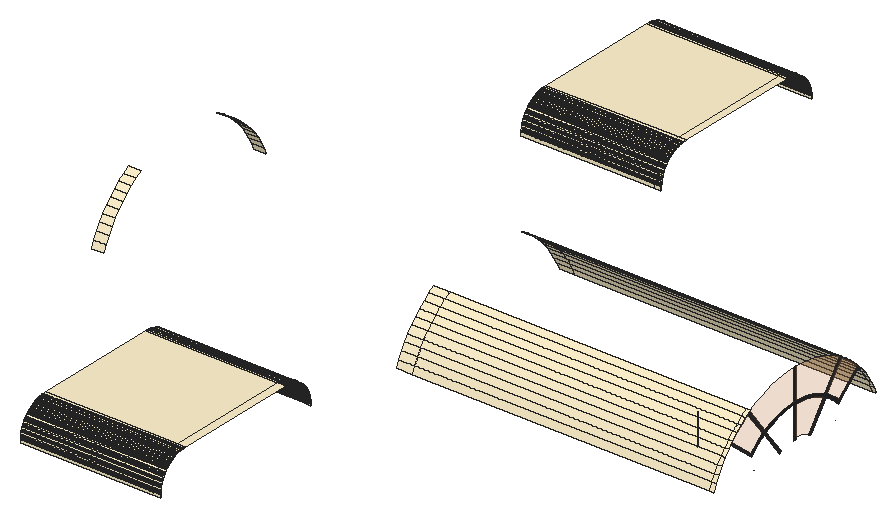
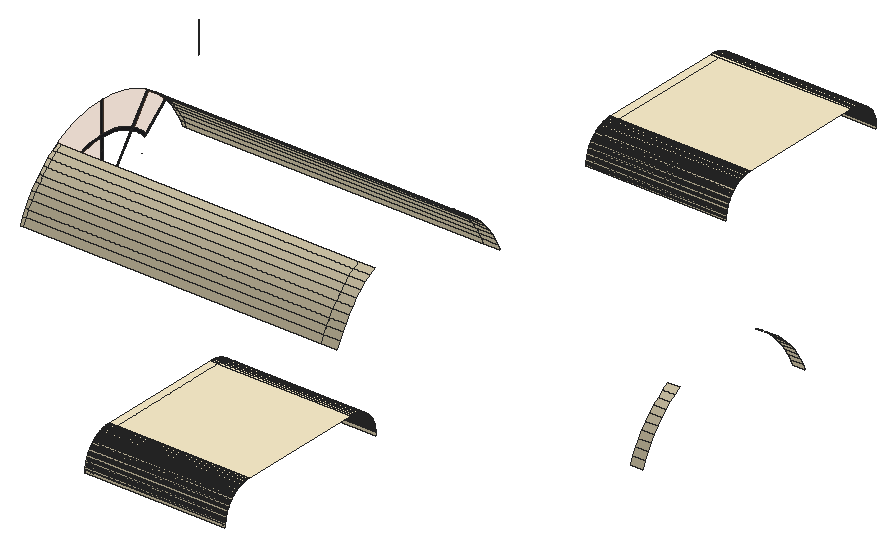
# SketchUp Ruby script. Lengths in inches.
U = 1.inch
M = Sketchup.active_model
def pt(a) = Geom::Point3d.new(a.map { |v| v * U })
def face(e, loops, mat)
  f = e.add_face(loops[0].map { |a| pt(a) })
  loops[1..].each { |l| e.add_face(l.map { |a| pt(a) }).erase! }
  f.material = f.back_material = mat if mat
  f
end
# faces: each face lists its corners as indices into pts; further lists are holes
def faces(e, pts, list, mat = nil) = list.each { |f| face(e, (f[0].is_a?(Array) ? f : [f]).map { |l| l.map { |i| pts[i] } }, mat) }
# xy, xz, yz: faces in a plane at the given z, y or x. An outline is a flat list of corners, or four numbers for a rectangle; further outlines are holes
def ring(l) = l.size == 4 ? [[l[0], l[1]], [l[2], l[1]], [l[2], l[3]], [l[0], l[3]]] : l.each_slice(2).to_a
def flat(e, list, mat, &to3) = list.each { |f| face(e, (f[0].is_a?(Array) ? f : [f]).map { |l| ring(l).map { |u, v| to3.(u, v) } }, mat) }
def xy(e, z, list, mat = nil) = flat(e, list, mat) { |x, y| [x, y, z] }
def xz(e, y, list, mat = nil) = flat(e, list, mat) { |x, z| [x, y, z] }
def yz(e, x, list, mat = nil) = flat(e, list, mat) { |y, z| [x, y, z] }
def lines(e, pts, list) = list.each { |a, b| e.add_line(pt(pts[a]), pt(pts[b])) }
# prism: a flat outline (further loops are holes) pulled along v
def prism(e, loops, v, mat = nil)
  f = face(e, loops, mat); d = Geom::Vector3d.new(v.map { |x| x * U })
  f.pushpull(f.normal.samedirection?(d) ? d.length : -d.length)
end
def box(e, o, s, mat = nil) = prism(e, [[o, [o[0] + s[0], o[1], o[2]], [o[0] + s[0], o[1] + s[1], o[2]], [o[0], o[1] + s[1], o[2]]]], [0, 0, s[2]], mat)
def at(x, y, z, deg = 0) = Geom::Transformation.translation(pt([x, y, z])) * Geom::Transformation.rotation(ORIGIN, Z_AXIS, deg.degrees)
def axes(o, x, y, z) = Geom::Transformation.new([*x, 0, *y, 0, *z, 0, *pt(o).to_a, 1])
def part(name) = M.definitions.add(name)
# library, detail: a bought-in or finely detailed component or shape, given as its bounding box
def library(name, o, s) = part(name).tap { |d| box(d.entities, o, s) }
def detail(e, o, s) = box(e.add_group.entities, o, s)
def put(e, d, t, mat = nil) = e.add_instance(d, t).tap { |i| i.material = mat if mat }
def group(e, t, mat = nil) = e.add_group.tap { |g| g.transformation = t; g.material = mat if mat }.entities
root = M.entities
M.materials.add("D01_Frost_White").color = [255, 242, 206]
M.materials.add("Glass_Safety_01").color = [244, 153, 81]
M.materials["Glass_Safety_01"].alpha = 0.25
M.materials.add("ThomThom - Buttons1").color = [48, 49, 53]
M.materials.add("ThomThom - Buttons2").color = [40, 40, 43]
xy(root,342,[[144.65,88.1,246,90],[246,88.1,252,90],[144.65,90,246,186],[246,90,252,186],[144.65,186,246,187.16],
  [246,186,252,187.16],[144.65,567.32,246,570],[246,567.32,252,570],[144.65,570,246,666],[246,570,252,666],
  [144.65,666,246,667.87],[246,666,252,667.87]],"D01_Frost_White")
xz(root,66,[[144.65,318,246,319.9],[246,318,252,319.9]],"D01_Frost_White")
xz(root,210,[[144.65,318,246,319.16],[246,318,252,319.16]],"D01_Frost_White")
xz(root,546,[[144.65,318,246,320.68],[246,318,252,320.68]],"D01_Frost_White")
xz(root,690,[[144.65,318,246,319.87],[246,318,252,319.87]],"D01_Frost_White")
yz(root,252,[[66,318,66,319.9,65.98,319.53,65.98,318.76],[210,318,210.01,318.76,210,319.16],[546,318,546,320.68,545.98,320.3,545.96,319.53,545.97,318.77],[690,318,690.02,318.76,690.01,319.53,690,319.87],[88.1,342,90,342,89.24,342.02,88.47,342.02],
  [186,342,187.16,342,186.76,342.01],[567.32,342,570,342,569.23,342.03,568.47,342.04,567.7,342.02],[666,342,667.87,342,667.53,342.01,666.76,342.02]],"D01_Frost_White")
yz(root,489,[[338.87,299.58,338.96,299.71,338.92,299.66],[417.13,299.58,417.08,299.66,417.04,299.71],[390.99,301.79,405.47,321.06,403.79,321.96,400.3125,323.54,396.74,324.89,393.09,325.99,389.375,326.86,385.61,327.49,381.8125,327.86,379,327.95,379,304.66,379.92,304.63,381.82,304.45,383.72,304.15,385.59,303.73,387.43,303.2,389.23,302.55],[419.56,310.51,419.21,310.875,418.48,311.56],[335.88,312.77,338.25,314.99,341.29,317.5,344.5,319.8,347.51,321.68,333.04,340.94,331.13,339.75,326.65,336.53,322.39,333.02,318.36,329.24,317.4,328.21],
  [420.03,312.85,438.53,328.29,437.64,329.24,433.61,333.02,429.35,336.53,424.87,339.75,422.83,341.02,422.26,340.27,408.36,321.76,411.5,319.8,414.71,317.5,417.75,314.99],[349.18,322.6,351.33,323.75,354.92,325.39,358.61,326.78,362.39,327.93,366.23,328.83,370.13,329.47,374.06,329.86,378,329.99,377,329.99,377,353.97,372.48,353.82,366.99,353.28,361.54,352.375,356.16,351.12,350.88,349.51,345.71,347.5625,340.6875,345.28,335.82,342.67,334.65,341.94],[406.68,322.68,421.22,342.02,420.18,342.67,415.3125,345.28,410.29,347.5625,405.12,349.51,399.84,351.12,394.46,352.375,389.01,353.28,383.52,353.82,379,353.97,379,329.99,378,329.99,381.94,329.86,385.87,329.47,389.77,328.83,393.61,327.93,397.39,326.78,401.08,325.39,404.67,323.75]],"Glass_Safety_01")
yz(root,489,[[363.12,300.92,364.82,301.79,350.4,320.99,348.85,320.16,348.72,320.08],[392.69,300.92,407.15,320.16,405.47,321.06,390.99,301.79],[336.36,310.42,336.79,310.875,337.43,311.47,337.32,311.56,336.25,310.51],[334.82,311.7,335.37,312.29,335.88,312.77,317.4,328.21,316.37,327.1],[421.1,311.79,439.55,327.19,438.53,328.29,420.03,312.85,420.63,312.29],
  [347.51,321.68,347.85,321.89,349.18,322.6,334.65,341.94,333.04,340.94],[408.36,321.76,422.26,340.27,422.83,341.02,421.22,342.02,406.68,322.68,408.15,321.89]],"ThomThom - Buttons1")
yz(root,489,[[377,303.66,378,303.6875,379,303.66,379,304.66,378,304.6875,377,304.66],[377,304.66,378,304.6875,379,304.66,379,319.07,378,319.08,377,319.07],[336.25,310.51,337.32,311.56,335.88,312.77,335.37,312.29,334.82,311.7],[419.56,310.51,421.1,311.79,420.63,312.29,420.03,312.85,418.48,311.56,419.21,310.875],[337.43,311.47,339.57,313.49,342.51,315.91,345.61,318.14,348.72,320.08,348.66,320.16,347.51,321.68,344.5,319.8,341.29,317.5,338.25,314.99,335.88,312.77,337.32,311.56],
  [418.48,311.56,420.03,312.85,417.75,314.99,414.71,317.5,411.5,319.8,408.36,321.76,407.15,320.16,410.39,318.14,413.49,315.91,416.43,313.49],[377,319.07,378,319.08,379,319.07,379,327.95,381.8125,327.86,385.61,327.49,389.375,326.86,393.09,325.99,396.74,324.89,400.3125,323.54,403.79,321.96,405.47,321.06,406.68,322.68,404.67,323.75,401.08,325.39,397.39,326.78,393.61,327.93,389.77,328.83,385.87,329.47,381.94,329.86,378,329.99,374.06,329.86,370.13,329.47,366.23,328.83,362.39,327.93,358.61,326.78,354.92,325.39,351.33,323.75,349.18,322.6,350.34,321.06,350.4,320.99,352.21,321.96,355.6875,323.54,359.26,324.89,362.91,325.99,366.625,326.86,370.39,327.49,374.1875,327.86,377,327.95],[348.72,320.08,348.85,320.16,350.4,320.99,350.34,321.06,348.66,320.16],[348.66,320.16,350.34,321.06,349.18,322.6,347.85,321.89,347.51,321.68],[407.15,320.16,408.36,321.76,408.15,321.89,406.68,322.68,405.47,321.06],
  [377,329.99,379,329.99,379,353.97,378,354,377,353.97]],"ThomThom - Buttons2")
yz(root,491,[[282,342,282.07,342.73,282.07,365.93,282,366]],"D01_Frost_White")
p = [[21,302.4,306.86],[21,300.13,301.83],[12,300.13,301.83],[12,302.4,306.86],[258,302.4,306.86],[258,300.13,301.83],
  [246,300.13,301.83],[246,302.4,306.86],[486,302.4,306.86],[486,300.13,301.83],[489,302.4,306.86],[489,300.13,301.83],
  [21,455.87,301.83],[21,453.6,306.86],[12,453.6,306.86],[12,455.87,301.83],[258,455.87,301.83],[258,453.6,306.86],
  [246,453.6,306.86],[246,455.87,301.83],[486,455.87,301.83],[486,453.6,306.86],[489,455.87,301.83],[489,453.6,306.86],
  [21,304.99,311.74],[12,304.99,311.74],[258,304.99,311.74],[246,304.99,311.74],[486,304.99,311.74],[489,304.99,311.74],
  [21,451.01,311.74],[12,451.01,311.74],[258,451.01,311.74],[246,451.01,311.74],[486,451.01,311.74],[489,451.01,311.74],
  [21,307.89,316.43],[12,307.89,316.43],[258,307.89,316.43],[246,307.89,316.43],[486,307.89,316.43],[489,307.89,316.43],
  [21,448.11,316.43],[12,448.11,316.43],[258,448.11,316.43],[246,448.11,316.43],[486,448.11,316.43],[489,448.11,316.43],
  [21,311.1,320.93],[12,311.1,320.93],[258,311.1,320.93],[246,311.1,320.93],[486,311.1,320.93],[489,311.1,320.93],
  [21,444.9,320.93],[12,444.9,320.93],[258,444.9,320.93],[246,444.9,320.93],[486,444.9,320.93],[489,444.9,320.93],
  [246,210,319.16],[246,209.99,319.52],[144.65,209.99,319.52],[144.65,210,319.16],[252,210,319.16],[252,209.99,319.52],
  [246,209.95,320.28],[144.65,209.95,320.28],[252,209.95,320.28],[246,66.02,320.29],[246,66,319.9],[144.65,66,319.9],
  [144.65,66.02,320.29],[252,66.02,320.29],[252,66,319.9],[246,690,319.87],[246,689.98,320.29],[144.65,689.98,320.29],
  [144.65,690,319.87],[252,690,319.87],[252,689.98,320.29],[246,66.07,321.05],[144.65,66.07,321.05],[252,66.07,321.05],
  [246,209.89,321.03],[144.65,209.89,321.03],[252,209.89,321.03],[246,689.93,321.05],[144.65,689.93,321.05],[252,689.93,321.05],
  [246,546.02,321.07],[246,546,320.68],[144.65,546,320.68],[144.65,546.02,321.07],[252,546.02,321.07],[252,546,320.68],
  [21,314.59,325.2],[12,314.59,325.2],[258,314.59,325.2],[246,314.59,325.2],[486,314.59,325.2],[489,314.59,325.2],
  [21,441.41,325.2],[12,441.41,325.2],[258,441.41,325.2],[246,441.41,325.2],[486,441.41,325.2],[489,441.41,325.2],
  [246,66.15,321.81],[144.65,66.15,321.81],[252,66.15,321.81],[246,209.8,321.79],[144.65,209.8,321.79],[252,209.8,321.79],
  [246,689.85,321.81],[144.65,689.85,321.81],[252,689.85,321.81],[246,546.09,321.83],[144.65,546.09,321.83],[252,546.09,321.83],
  [246,66.26,322.5625],[144.65,66.26,322.5625],[252,66.26,322.5625],[246,209.68,322.54],[144.65,209.68,322.54],[252,209.68,322.54],
  [246,546.1875,322.59],[144.65,546.1875,322.59],[252,546.1875,322.59],[246,689.74,322.5625],[144.65,689.74,322.5625],[252,689.74,322.5625],
  [246,209.54,323.29],[144.65,209.54,323.29],[252,209.54,323.29],[246,66.39,323.32],[144.65,66.39,323.32],[252,66.39,323.32],
  [246,546.3125,323.35],[144.65,546.3125,323.35],[252,546.3125,323.35],[246,689.61,323.31],[144.65,689.61,323.31],[252,689.61,323.31],
  [246,66.54,324.0625],[144.65,66.54,324.0625],[252,66.54,324.0625],[246,209.38,324.03],[144.65,209.38,324.03],[252,209.38,324.03],
  [246,546.46,324.1],[144.65,546.46,324.1],[252,546.46,324.1],[246,689.45,324.0625],[144.65,689.45,324.0625],[252,689.45,324.0625],
  [246,209.19,324.77],[144.65,209.19,324.77],[252,209.19,324.77],[246,66.72,324.8],[144.65,66.72,324.8],[252,66.72,324.8],
  [246,546.63,324.85],[144.65,546.63,324.85],[252,546.63,324.85],[246,689.27,324.8],[144.65,689.27,324.8],[252,689.27,324.8],
  [246,66.93,325.54],[144.65,66.93,325.54],[252,66.93,325.54],[246,208.98,325.5],[144.65,208.98,325.5],[252,208.98,325.5],
  [246,546.83,325.59],[144.65,546.83,325.59],[252,546.83,325.59],[246,689.07,325.54],[144.65,689.07,325.54],[252,689.07,325.54],
  [21,318.36,329.24],[12,318.36,329.24],[258,318.36,329.24],[246,318.36,329.24],[486,318.36,329.24],[489,316.37,327.1],
  [489,318.36,329.24],[489,317.4,328.21],[21,437.64,329.24],[12,437.64,329.24],[258,437.64,329.24],[246,437.64,329.24],
  [486,437.64,329.24],[489,438.53,328.29],[489,437.64,329.24],[489,439.55,327.19],[246,67.16,326.27],[144.65,67.16,326.27],
  [252,67.16,326.27],[246,208.75,326.22],[144.65,208.75,326.22],[252,208.75,326.22],[246,688.84,326.27],[144.65,688.84,326.27],
  [252,688.84,326.27],[246,547.05,326.32],[144.65,547.05,326.32],[252,547.05,326.32],[246,208.49,326.93],[144.65,208.49,326.93],
  [252,208.49,326.93],[246,67.41,326.99],[144.65,67.41,326.99],[252,67.41,326.99],[246,547.3,327.05],[144.65,547.3,327.05],
  [252,547.3,327.05],[246,688.58,326.98],[144.65,688.58,326.98],[252,688.58,326.98],[246,208.21,327.64],[144.65,208.21,327.64],
  [252,208.21,327.64],[246,67.6875,327.7],[144.65,67.6875,327.7],[252,67.6875,327.7],[246,547.57,327.77],[144.65,547.57,327.77],
  [252,547.57,327.77],[246,688.31,327.7],[144.65,688.31,327.7],[252,688.31,327.7],[246,207.9,328.33],[144.65,207.9,328.33],
  [252,207.9,328.33],[246,67.99,328.4],[144.65,67.99,328.4],[252,67.99,328.4],[246,688.01,328.4],[144.65,688.01,328.4],
  [252,688.01,328.4],[246,547.87,328.47],[144.65,547.87,328.47],[252,547.87,328.47],[246,207.58,329.02],[144.65,207.58,329.02],
  [252,207.58,329.02],[246,68.3125,329.09],[144.65,68.3125,329.09],[252,68.3125,329.09],[246,687.68,329.09],[144.65,687.68,329.09],
  [252,687.68,329.09],[246,548.1875,329.17],[144.65,548.1875,329.17],[252,548.1875,329.17],[246,207.23,329.7],[144.65,207.23,329.7],
  [252,207.23,329.7],[246,68.66,329.77],[144.65,68.66,329.77],[252,68.66,329.77],[246,687.34,329.77],[144.65,687.34,329.77],
  [252,687.34,329.77],[21,322.39,333.02],[12,322.39,333.02],[258,322.39,333.02],[246,322.39,333.02],[486,322.39,333.02],
  [489,322.39,333.02],[21,433.61,333.02],[12,433.61,333.02],[258,433.61,333.02],[246,433.61,333.02],[486,433.61,333.02],
  [489,433.61,333.02],[246,548.53,329.86],[144.65,548.53,329.86],[252,548.53,329.86],[246,206.86,330.36],[144.65,206.86,330.36],
  [252,206.86,330.36],[246,69.03,330.44],[144.65,69.03,330.44],[252,69.03,330.44],[246,686.97,330.4375],[144.65,686.97,330.4375],
  [252,686.97,330.4375],[246,548.9,330.53],[144.65,548.9,330.53],[252,548.9,330.53],[246,69.42,331.1],[144.65,69.42,331.1],
  [252,69.42,331.1],[246,206.47,331.01],[144.65,206.47,331.01],[252,206.47,331.01],[246,686.58,331.09],[144.65,686.58,331.09],
  [252,686.58,331.09],[246,549.29,331.19],[144.65,549.29,331.19],[252,549.29,331.19],[246,206.05,331.65],[144.65,206.05,331.65],
  [252,206.05,331.65],[246,69.83,331.74],[144.65,69.83,331.74],[252,69.83,331.74],[246,686.17,331.73],[144.65,686.17,331.73],
  [252,686.17,331.73],[246,549.7,331.84],[144.65,549.7,331.84],[252,549.7,331.84],[246,205.62,332.27],[144.65,205.62,332.27],
  [252,205.62,332.27],[246,70.26,332.37],[144.65,70.26,332.37],[252,70.26,332.37],[246,685.73,332.36],[144.65,685.73,332.36],
  [252,685.73,332.36],[246,550.13,332.47],[144.65,550.13,332.47],[252,550.13,332.47],[246,205.17,332.88],[144.65,205.17,332.88],
  [252,205.17,332.88],[246,70.71,332.98],[144.65,70.71,332.98],[252,70.71,332.98],[246,685.28,332.98],[144.65,685.28,332.98],
  [252,685.28,332.98],[246,550.58,333.09],[144.65,550.58,333.09],[252,550.58,333.09],[246,204.69,333.48],[144.65,204.69,333.48],
  [252,204.69,333.48],[246,71.1875,333.58],[144.65,71.1875,333.58],[252,71.1875,333.58],[21,326.65,336.53],[12,326.65,336.53],
  [258,326.65,336.53],[246,326.65,336.53],[486,326.65,336.53],[489,326.65,336.53],[21,429.35,336.53],[12,429.35,336.53],
  [258,429.35,336.53],[246,429.35,336.53],[486,429.35,336.53],[489,429.35,336.53],[246,684.81,333.57],[144.65,684.81,333.57],
  [252,684.81,333.57],[246,551.06,333.69],[144.65,551.06,333.69],[252,551.06,333.69],[246,204.2,334.06],[144.65,204.2,334.06],
  [252,204.2,334.06],[246,71.68,334.16],[144.65,71.68,334.16],[252,71.68,334.16],[246,684.3125,334.16],[144.65,684.3125,334.16],
  [252,684.3125,334.16],[246,551.55,334.28],[144.65,551.55,334.28],[252,551.55,334.28],[246,203.69,334.62],[144.65,203.69,334.62],
  [252,203.69,334.62],[246,72.19,334.73],[144.65,72.19,334.73],[252,72.19,334.73],[246,683.8,334.72],[144.65,683.8,334.72],
  [252,683.8,334.72],[246,552.07,334.85],[144.65,552.07,334.85],[252,552.07,334.85],[246,203.16,335.16],[144.65,203.16,335.16],
  [252,203.16,335.16],[246,72.72,335.28],[144.65,72.72,335.28],[252,72.72,335.28],[246,683.27,335.27],[144.65,683.27,335.27],
  [252,683.27,335.27],[246,552.6,335.4],[144.65,552.6,335.4],[252,552.6,335.4],[246,202.62,335.69],[144.65,202.62,335.69],
  [252,202.62,335.69],[246,73.27,335.81],[144.65,73.27,335.81],[252,73.27,335.81],[246,682.72,335.8],[144.65,682.72,335.8],
  [252,682.72,335.8],[246,553.15,335.93],[144.65,553.15,335.93],[252,553.15,335.93],[246,202.06,336.2],[144.65,202.06,336.2],
  [252,202.06,336.2],[246,73.84,336.32],[144.65,73.84,336.32],[252,73.84,336.32],[246,682.16,336.3125],[144.65,682.16,336.3125],
  [252,682.16,336.3125],[246,553.72,336.45],[144.65,553.72,336.45],[252,553.72,336.45],[246,201.48,336.69],[144.65,201.48,336.69],
  [252,201.48,336.69],[246,74.42,336.8125],[144.65,74.42,336.8125],[252,74.42,336.8125],[246,681.57,336.81],[144.65,681.57,336.81],
  [252,681.57,336.81],[246,554.31,336.94],[144.65,554.31,336.94],[252,554.31,336.94],[21,331.13,339.75],[12,331.13,339.75],
  [258,331.13,339.75],[246,331.13,339.75],[486,331.13,339.75],[489,331.13,339.75],[21,424.87,339.75],[12,424.87,339.75],
  [258,424.87,339.75],[246,424.87,339.75],[486,424.87,339.75],[489,424.87,339.75],[246,200.88,337.17],[144.65,200.88,337.17],
  [252,200.88,337.17],[246,75.02,337.29],[144.65,75.02,337.29],[252,75.02,337.29],[246,680.98,337.28],[144.65,680.98,337.28],
  [252,680.98,337.28],[246,554.91,337.42],[144.65,554.91,337.42],[252,554.91,337.42],[246,200.27,337.62],[144.65,200.27,337.62],
  [252,200.27,337.62],[246,75.63,337.74],[144.65,75.63,337.74],[252,75.63,337.74],[246,680.36,337.73],[144.65,680.36,337.73],
  [252,680.36,337.73],[246,555.53,337.87],[144.65,555.53,337.87],[252,555.53,337.87],[246,199.65,338.05],[144.65,199.65,338.05],
  [252,199.65,338.05],[246,76.26,338.17],[144.65,76.26,338.17],[252,76.26,338.17],[246,679.73,338.17],[144.65,679.73,338.17],
  [252,679.73,338.17],[246,556.16,338.3],[144.65,556.16,338.3],[252,556.16,338.3],[246,199.01,338.47],[144.65,199.01,338.47],
  [252,199.01,338.47],[246,76.9,338.58],[144.65,76.9,338.58],[252,76.9,338.58],[246,679.09,338.58],[144.65,679.09,338.58],
  [252,679.09,338.58],[246,556.81,338.71],[144.65,556.81,338.71],[252,556.81,338.71],[246,198.36,338.86],[144.65,198.36,338.86],
  [252,198.36,338.86],[246,77.56,338.97],[144.65,77.56,338.97],[252,77.56,338.97],[246,678.4375,338.97],[144.65,678.4375,338.97],
  [252,678.4375,338.97],[246,557.47,339.1],[144.65,557.47,339.1],[252,557.47,339.1],[246,197.7,339.23],[144.65,197.7,339.23],
  [252,197.7,339.23],[246,78.23,339.34],[144.65,78.23,339.34],[252,78.23,339.34],[246,677.77,339.34],[144.65,677.77,339.34],
  [252,677.77,339.34],[246,558.14,339.47],[144.65,558.14,339.47],[252,558.14,339.47],[246,197.02,339.58],[144.65,197.02,339.58],
  [252,197.02,339.58],[246,78.91,339.6875],[144.65,78.91,339.6875],[252,78.91,339.6875],[246,677.09,339.68],[144.65,677.09,339.68],
  [252,677.09,339.68],[246,558.83,339.8125],[144.65,558.83,339.8125],[252,558.83,339.8125],[246,196.33,339.9],[144.65,196.33,339.9],
  [252,196.33,339.9],[246,79.6,340.01],[144.65,79.6,340.01],[252,79.6,340.01],[246,676.4,340.01],[144.65,676.4,340.01],
  [252,676.4,340.01],[21,335.82,342.67],[12,335.82,342.67],[258,335.82,342.67],[246,335.82,342.67],[486,335.82,342.67],
  [489,333.04,340.94],[489,335.82,342.67],[489,334.65,341.94],[21,420.18,342.67],[12,420.18,342.67],[258,420.18,342.67],
  [246,420.18,342.67],[486,420.18,342.67],[489,421.22,342.02],[489,420.18,342.67],[489,422.83,341.02],[246,559.53,340.13],
  [144.65,559.53,340.13],[252,559.53,340.13],[246,195.64,340.21],[144.65,195.64,340.21],[252,195.64,340.21],[246,80.3,340.3125],
  [144.65,80.3,340.3125],[252,80.3,340.3125],[246,675.7,340.31],[144.65,675.7,340.31],[252,675.7,340.31],[246,560.23,340.43],
  [144.65,560.23,340.43],[252,560.23,340.43],[246,194.93,340.49],[144.65,194.93,340.49],[252,194.93,340.49],[246,81.01,340.59],
  [144.65,81.01,340.59],[252,81.01,340.59],[246,674.98,340.58],[144.65,674.98,340.58],[252,674.98,340.58],[246,560.95,340.7],
  [144.65,560.95,340.7],[252,560.95,340.7],[246,194.22,340.75],[144.65,194.22,340.75],[252,194.22,340.75],[246,81.73,340.84],
  [144.65,81.73,340.84],[252,81.73,340.84],[246,674.27,340.84],[144.65,674.27,340.84],[252,674.27,340.84],[246,193.5,340.98],
  [144.65,193.5,340.98],[252,193.5,340.98],[246,561.68,340.95],[144.65,561.68,340.95],[252,561.68,340.95],[246,82.46,341.07],
  [144.65,82.46,341.07],[252,82.46,341.07],[246,673.54,341.07],[144.65,673.54,341.07],[252,673.54,341.07],[246,562.41,341.17],
  [144.65,562.41,341.17],[252,562.41,341.17],[246,192.77,341.19],[144.65,192.77,341.19],[252,192.77,341.19],[246,83.2,341.28],
  [144.65,83.2,341.28],[252,83.2,341.28],[246,672.8,341.27],[144.65,672.8,341.27],[252,672.8,341.27],[246,192.03,341.38],
  [144.65,192.03,341.38],[252,192.03,341.38],[246,563.15,341.37],[144.65,563.15,341.37],[252,563.15,341.37],[246,83.9375,341.46],
  [144.65,83.9375,341.46],[252,83.9375,341.46],[246,672.0625,341.45],[144.65,672.0625,341.45],[252,672.0625,341.45],[246,191.29,341.54],
  [144.65,191.29,341.54],[252,191.29,341.54],[246,563.9,341.54],[144.65,563.9,341.54],[252,563.9,341.54],[246,84.68,341.61],
  [144.65,84.68,341.61],[252,84.68,341.61],[246,190.54,341.68],[144.65,190.54,341.68],[252,190.54,341.68],[246,564.65,341.6875],
  [144.65,564.65,341.6875],[252,564.65,341.6875],[246,671.31,341.61],[144.65,671.31,341.61],[252,671.31,341.61],[246,85.4375,341.74],
  [144.65,85.4375,341.74],[252,85.4375,341.74],[246,670.5625,341.74],[144.65,670.5625,341.74],[252,670.5625,341.74],[246,86.19,341.85],
  [144.65,86.19,341.85],[252,86.19,341.85],[246,189.79,341.8],[144.65,189.79,341.8],[252,189.79,341.8],[246,565.41,341.8125],
  [144.65,565.41,341.8125],[252,565.41,341.8125],[246,669.81,341.85],[144.65,669.81,341.85],[252,669.81,341.85],[246,86.95,341.93],
  [144.65,86.95,341.93],[252,86.95,341.93],[246,189.03,341.89],[144.65,189.03,341.89],[252,189.03,341.89],[246,566.17,341.91],
  [144.65,566.17,341.91],[252,566.17,341.91],[246,669.05,341.93],[144.65,669.05,341.93],[252,669.05,341.93],[246,87.71,341.98],
  [144.65,87.71,341.98],[252,87.71,341.98],[246,188.28,341.95],[144.65,188.28,341.95],[252,188.28,341.95],[246,566.93,341.98],
  [144.65,566.93,341.98],[252,566.93,341.98],[246,668.29,341.98],[144.65,668.29,341.98],[252,668.29,341.98],[246,88.1,342],
  [144.65,88.1,342],[252,88.1,342],[246,187.52,341.99],[246,187.16,342],[144.65,187.16,342],[144.65,187.52,341.99],
  [252,187.52,341.99],[252,187.16,342],[246,567.32,342],[144.65,567.32,342],[252,567.32,342],[246,667.87,342],
  [144.65,667.87,342],[252,667.87,342],[489,379,327.99],[489,379,327.95],[489,377,327.99],[489,377,327.95]]
faces(root,p,[[0,1,2,3],[4,5,6,7],[8,9,5,4],[10,11,9,8],[12,13,14,15],[16,17,18,19],[20,21,17,16],[22,23,21,20],
  [24,0,3,25],[26,4,7,27],[28,8,4,26],[29,10,8,28],[13,30,31,14],[17,32,33,18],[21,34,32,17],[23,35,34,21],
  [36,24,25,37],[38,26,27,39],[40,28,26,38],[41,29,28,40],[30,42,43,31],[32,44,45,33],[34,46,44,32],[35,47,46,34],
  [48,36,37,49],[50,38,39,51],[52,40,38,50],[53,41,40,52],[42,54,55,43],[44,56,57,45],[46,58,56,44],[47,59,58,46],
  [60,61,62,63],[64,65,61,60],[61,66,67,62],[65,68,66,61],[69,70,71,72],[73,74,70,69],[75,76,77,78],[79,80,76,75],
  [81,69,72,82],[83,73,69,81],[66,84,85,67],[68,86,84,66],[76,87,88,77],[80,89,87,76],[90,91,92,93],[94,95,91,90],
  [96,48,49,97],[98,50,51,99],[100,52,50,98],[101,53,52,100],[54,102,103,55],[56,104,105,57],[58,106,104,56],[59,107,106,58],
  [108,81,82,109],[110,83,81,108],[84,111,112,85],[86,113,111,84],[87,114,115,88],[89,116,114,87],[117,90,93,118],[119,94,90,117],
  [120,108,109,121],[122,110,108,120],[111,123,124,112],[113,125,123,111],[126,117,118,127],[128,119,117,126],[114,129,130,115],[116,131,129,114],
  [123,132,133,124],[125,134,132,123],[135,120,121,136],[137,122,120,135],[138,126,127,139],[140,128,126,138],[129,141,142,130],[131,143,141,129],
  [144,135,136,145],[146,137,135,144],[132,147,148,133],[134,149,147,132],[150,138,139,151],[152,140,138,150],[141,153,154,142],[143,155,153,141],
  [147,156,157,148],[149,158,156,147],[159,144,145,160],[161,146,144,159],[162,150,151,163],[164,152,150,162],[153,165,166,154],[155,167,165,153],
  [168,159,160,169],[170,161,159,168],[156,171,172,157],[158,173,171,156],[174,162,163,175],[176,164,162,174],[165,177,178,166],[167,179,177,165],
  [180,96,97,181],[182,98,99,183],[184,100,98,182],[185,101,100,184,186,187],[102,188,189,103],[104,190,191,105],[106,192,190,104],[193,194,192,106,107,195],
  [196,168,169,197],[198,170,168,196],[171,199,200,172],[173,201,199,171],[177,202,203,178],[179,204,202,177],[205,174,175,206],[207,176,174,205],
  [199,208,209,200],[201,210,208,199],[211,196,197,212],[213,198,196,211],[214,205,206,215],[216,207,205,214],[202,217,218,203],[204,219,217,202],
  [208,220,221,209],[210,222,220,208],[223,211,212,224],[225,213,211,223],[226,214,215,227],[228,216,214,226],[217,229,230,218],[219,231,229,217],
  [220,232,233,221],[222,234,232,220],[235,223,224,236],[237,225,223,235],[229,238,239,230],[231,240,238,229],[241,226,227,242],[243,228,226,241],
  [232,244,245,233],[234,246,244,232],[247,235,236,248],[249,237,235,247],[238,250,251,239],[240,252,250,238],[253,241,242,254],[255,243,241,253],
  [244,256,257,245],[246,258,256,244],[259,247,248,260],[261,249,247,259],[250,262,263,251],[252,264,262,250],[265,180,181,266],[267,182,183,268],
  [269,184,182,267],[270,186,184,269],[188,271,272,189],[190,273,274,191],[192,275,273,190],[194,276,275,192],[277,253,254,278],[279,255,253,277],
  [256,280,281,257],[258,282,280,256],[283,259,260,284],[285,261,259,283],[262,286,287,263],[264,288,286,262],[289,277,278,290],[291,279,277,289],
  [292,283,284,293],[294,285,283,292],[280,295,296,281],[282,297,295,280],[286,298,299,287],[288,300,298,286],[301,289,290,302],[303,291,289,301],
  [295,304,305,296],[297,306,304,295],[307,292,293,308],[309,294,292,307],[298,310,311,299],[300,312,310,298],[313,301,302,314],[315,303,301,313],
  [304,316,317,305],[306,318,316,304],[319,307,308,320],[321,309,307,319],[310,322,323,311],[312,324,322,310],[325,313,314,326],[327,315,313,325],
  [316,328,329,317],[318,330,328,316],[331,319,320,332],[333,321,319,331],[322,334,335,323],[324,336,334,322],[337,325,326,338],[339,327,325,337],
  [328,340,341,329],[330,342,340,328],[343,331,332,344],[345,333,331,343],[346,265,266,347],[348,267,268,349],[350,269,267,348],[351,270,269,350],
  [271,352,353,272],[273,354,355,274],[275,356,354,273],[276,357,356,275],[334,358,359,335],[336,360,358,334],[361,337,338,362],[363,339,337,361],
  [340,364,365,341],[342,366,364,340],[367,343,344,368],[369,345,343,367],[358,370,371,359],[360,372,370,358],[373,361,362,374],[375,363,361,373],
  [364,376,377,365],[366,378,376,364],[379,367,368,380],[381,369,367,379],[370,382,383,371],[372,384,382,370],[385,373,374,386],[387,375,373,385],
  [376,388,389,377],[378,390,388,376],[391,379,380,392],[393,381,379,391],[382,394,395,383],[384,396,394,382],[397,385,386,398],[399,387,385,397],
  [388,400,401,389],[390,402,400,388],[403,391,392,404],[405,393,391,403],[394,406,407,395],[396,408,406,394],[409,397,398,410],[411,399,397,409],
  [400,412,413,401],[402,414,412,400],[415,403,404,416],[417,405,403,415],[406,418,419,407],[408,420,418,406],[421,409,410,422],[423,411,409,421],
  [412,424,425,413],[414,426,424,412],[427,415,416,428],[429,417,415,427],[418,430,431,419],[420,432,430,418],[433,421,422,434],[435,423,421,433],
  [436,346,347,437],[438,348,349,439],[440,350,348,438],[441,351,350,440],[352,442,443,353],[354,444,445,355],[356,446,444,354],[357,447,446,356],
  [424,448,449,425],[426,450,448,424],[451,427,428,452],[453,429,427,451],[430,454,455,431],[432,456,454,430],[457,433,434,458],[459,435,433,457],
  [448,460,461,449],[450,462,460,448],[463,451,452,464],[465,453,451,463],[454,466,467,455],[456,468,466,454],[469,457,458,470],[471,459,457,469],
  [460,472,473,461],[462,474,472,460],[475,463,464,476],[477,465,463,475],[466,478,479,467],[468,480,478,466],[481,469,470,482],[483,471,469,481],
  [472,484,485,473],[474,486,484,472],[487,475,476,488],[489,477,475,487],[478,490,491,479],[480,492,490,478],[493,481,482,494],[495,483,481,493],
  [484,496,497,485],[486,498,496,484],[499,487,488,500],[501,489,487,499],[490,502,503,491],[492,504,502,490],[505,493,494,506],[507,495,493,505],
  [496,508,509,497],[498,510,508,496],[511,499,500,512],[513,501,499,511],[502,514,515,503],[504,516,514,502],[517,505,506,518],[519,507,505,517],
  [508,520,521,509],[510,522,520,508],[523,511,512,524],[525,513,511,523],[514,526,527,515],[516,528,526,514],[529,517,518,530],[531,519,517,529],
  [520,532,533,521],[522,534,532,520],[535,523,524,536],[537,525,523,535],[526,538,539,527],[528,540,538,526],[541,436,437,542],[543,438,439,544],
  [545,440,438,543],[546,441,440,545,547,548],[442,549,550,443],[444,551,552,445],[446,553,551,444],[554,555,553,446,447,556],[557,529,530,558],[559,531,529,557],
  [532,560,561,533],[534,562,560,532],[563,535,536,564],[565,537,535,563],[538,566,567,539],[540,568,566,538],[569,557,558,570],[571,559,557,569],
  [560,572,573,561],[562,574,572,560],[575,563,564,576],[577,565,563,575],[566,578,579,567],[568,580,578,566],[581,569,570,582],[583,571,569,581],
  [572,584,585,573],[574,586,584,572],[587,575,576,588],[589,577,575,587],[578,590,591,579],[580,592,590,578],[584,593,594,585],[586,595,593,584],
  [596,581,582,597],[598,583,581,596],[599,587,588,600],[601,589,587,599],[590,602,603,591],[592,604,602,590],[605,596,597,606],[607,598,596,605],
  [593,608,609,594],[595,610,608,593],[611,599,600,612],[613,601,599,611],[602,614,615,603],[604,616,614,602],[608,617,618,609],[610,619,617,608],
  [620,605,606,621],[622,607,605,620],[623,611,612,624],[625,613,611,623],[614,626,627,615],[616,628,626,614],[617,629,630,618],[619,631,629,617],
  [632,620,621,633],[634,622,620,632],[635,623,624,636],[637,625,623,635],[629,638,639,630],[631,640,638,629],[641,632,633,642],[643,634,632,641],
  [626,644,645,627],[628,646,644,626],[647,635,636,648],[649,637,635,647],[644,650,651,645],[646,652,650,644],[653,647,648,654],[655,649,647,653],
  [638,656,657,639],[640,658,656,638],[659,641,642,660],[661,643,641,659],[650,662,663,651],[652,664,662,650],[665,653,654,666],[667,655,653,665],
  [656,668,669,657],[658,670,668,656],[671,659,660,672],[673,661,659,671],[662,674,675,663],[664,676,674,662],[677,665,666,678],[679,667,665,677],
  [668,680,681,669],[670,682,680,668],[683,671,672,684],[685,673,671,683],[674,686,687,675],[676,688,686,674],[689,677,678,690],[691,679,677,689],
  [692,693,694,695],[696,697,693,692],[680,692,695,681],[682,696,692,680],[698,683,684,699],[700,685,683,698],[686,701,702,687],[688,703,701,686]],"D01_Frost_White")
lines(root,p,[[704,705],[706,707]])
